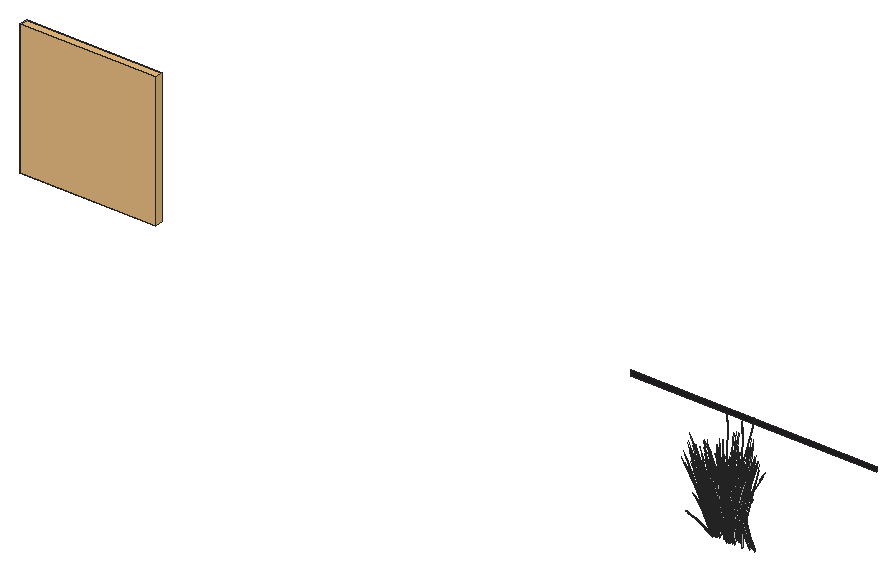
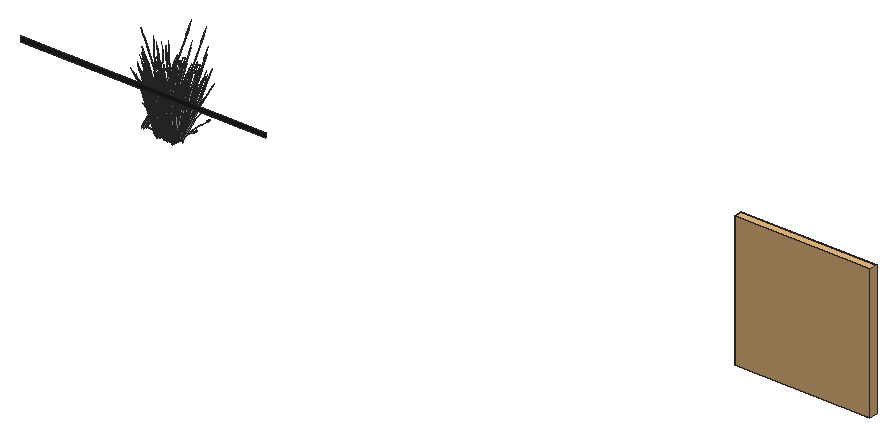
# SketchUp Ruby script. Lengths in inches.
U = 1.inch
M = Sketchup.active_model
def pt(a) = Geom::Point3d.new(a.map { |v| v * U })
def face(e, loops, mat)
  f = e.add_face(loops[0].map { |a| pt(a) })
  loops[1..].each { |l| e.add_face(l.map { |a| pt(a) }).erase! }
  f.material = f.back_material = mat if mat
  f
end
# faces: each face lists its corners as indices into pts; further lists are holes
def faces(e, pts, list, mat = nil) = list.each { |f| face(e, (f[0].is_a?(Array) ? f : [f]).map { |l| l.map { |i| pts[i] } }, mat) }
# xy, xz, yz: faces in a plane at the given z, y or x. An outline is a flat list of corners, or four numbers for a rectangle; further outlines are holes
def ring(l) = l.size == 4 ? [[l[0], l[1]], [l[2], l[1]], [l[2], l[3]], [l[0], l[3]]] : l.each_slice(2).to_a
def flat(e, list, mat, &to3) = list.each { |f| face(e, (f[0].is_a?(Array) ? f : [f]).map { |l| ring(l).map { |u, v| to3.(u, v) } }, mat) }
def xy(e, z, list, mat = nil) = flat(e, list, mat) { |x, y| [x, y, z] }
def xz(e, y, list, mat = nil) = flat(e, list, mat) { |x, z| [x, y, z] }
def yz(e, x, list, mat = nil) = flat(e, list, mat) { |y, z| [x, y, z] }
def lines(e, pts, list) = list.each { |a, b| e.add_line(pt(pts[a]), pt(pts[b])) }
# prism: a flat outline (further loops are holes) pulled along v
def prism(e, loops, v, mat = nil)
  f = face(e, loops, mat); d = Geom::Vector3d.new(v.map { |x| x * U })
  f.pushpull(f.normal.samedirection?(d) ? d.length : -d.length)
end
def box(e, o, s, mat = nil) = prism(e, [[o, [o[0] + s[0], o[1], o[2]], [o[0] + s[0], o[1] + s[1], o[2]], [o[0], o[1] + s[1], o[2]]]], [0, 0, s[2]], mat)
def at(x, y, z, deg = 0) = Geom::Transformation.translation(pt([x, y, z])) * Geom::Transformation.rotation(ORIGIN, Z_AXIS, deg.degrees)
def axes(o, x, y, z) = Geom::Transformation.new([*x, 0, *y, 0, *z, 0, *pt(o).to_a, 1])
def part(name) = M.definitions.add(name)
# library, detail: a bought-in or finely detailed component or shape, given as its bounding box
def library(name, o, s) = part(name).tap { |d| box(d.entities, o, s) }
def detail(e, o, s) = box(e.add_group.entities, o, s)
def put(e, d, t, mat = nil) = e.add_instance(d, t).tap { |i| i.material = mat if mat }
def group(e, t, mat = nil) = e.add_group.tap { |g| g.transformation = t; g.material = mat if mat }.entities
root = M.entities
M.materials.add("LightPink_Translucent").color = [144, 107, 117]
M.materials["LightPink_Translucent"].alpha = 0.75
M.materials.add("Marble_07_1K").color = [36, 34, 36]
c1 = library("mesh-163",[-551.08,-704.17,-20.03],[1929.24,1401.85,86.96])
c2 = part("Group11")
put(c2.entities,c1,at(0,0,0))
c3 = part("blade")
p = [[2.15,0.21,22],[0,0.17,0],[0.09,0.45,0],[2.18,0.31,22],[2.29,0.31,22],[0.38,0.45,0],
  [2.48,0.24,33],[2.49,0.24,33],[2.48,0.22,33]]
faces(c3.entities,p,[[0,1,2,3],[4,5,2,3],[6,3,4,7],[8,0,3,6]])
c4 = part("seeds")
p = [[0.3,-0.1,1.38],[-0.01,-0.03,1.59],[-0.01,-0.03,0.03],[0.14,-0.07,-0.07],[0.29,-0.03,3],[0.15,0.01,3.11]]
faces(c4.entities,p,[[0,1,2,3],[1,0,4,5]],"LightPink_Translucent")
c5 = part("blade with seeds")
put(c5.entities,c3,at(0,0,0))
put(c5.entities,c4,axes([2.4,0.25,30.99],[1.5799,-0.05474,1.17369],[-0.12525,1.92788,0.29478],[-0.07173,-0.02425,1.56792]))
xz(root,360,[[603,298,706,300]],"Marble_07_1K")
put(root,c2,axes([387.26,360.79,312.36],[-0.02948,0,0],[0,0,0.03987],[0,0.03937,0]))
put(root,c5,axes([657.47,336.1,267.22],[0.26985,-0.01293,1.42242],[-0.17902,0.56047,0.11501],[-0.38456,-0.03467,0.60807]))
put(root,c5,axes([657.58,337.08,267.22],[0.22574,-0.12077,1.42242],[0.19004,0.55807,0.11501],[-0.35439,0.12613,0.60807]))
put(root,c5,axes([658.875,336.5,266.77],[0.18493,-0.0826,1.46963],[0.06377,0.5767,0.11501],[-0.40056,0.07652,0.52526]))
put(root,c5,axes([656.89,336.89,267.91],[-0.10624,0.07413,1.45204],[0.00904,0.54162,-0.22964],[-0.24352,0.07044,0.11645]))
put(root,c5,axes([658.27,335.58,268.13],[-0.65035,-0.01375,-0.58968],[0.04368,-0.5789,0.07116],[-0.27552,-0.06109,0.83415]))
put(root,c5,axes([657.23,336.58,267.76],[-0.54068,-0.15928,-0.29394],[0.1577,-0.46469,0.37948],[-0.21769,0.04261,0.72609]))
put(root,c5,axes([655.71,337.43,267.91],[0.08303,0.01531,1.47228],[0.25685,0.50448,-0.13912],[-0.16996,0.13241,0.26054]))
put(root,c5,axes([657.6,336.8125,267.89],[-0.17625,0.51936,-0.42412],[-0.60429,-0.17802,-0.32852],[-0.2433,0.04762,0.81151]))
put(root,c5,axes([658.06,335.69,267.89],[-0.47241,0.37822,-0.42412],[-0.41372,-0.39954,-0.32852],[-0.24002,-0.05755,0.81151]))
put(root,c5,axes([657.39,334.63,267.91],[0.04823,0.05698,1.47228],[-0.23252,0.51221,-0.13912],[-0.23548,0.00371,0.26054]))
put(root,c5,axes([657.93,334.29,267.91],[-0.13998,-0.00403,1.45204],[-0.44565,0.40302,-0.22964],[-0.23779,-0.08235,0.11645]))
put(root,c5,axes([657.35,336.52,267.93],[0.18381,-0.5206,0.39842],[0.60429,0.17802,0.32852],[-0.23764,0.03129,0.82444]))
put(root,c5,axes([657.57,336.37,268.18],[0.32734,0.51701,-0.10093],[-0.58097,0.25407,-0.56021],[-0.24483,0.06821,0.85122]))
put(root,c5,axes([658.3,335.3,268.18],[-0.03484,0.58066,-0.10093],[-0.65957,-0.01587,-0.56021],[-0.25402,-0.04034,0.85122]))
put(root,c5,axes([657.88,335.34,267.76],[-0.37017,-0.35748,-0.29394],[0.42268,-0.3384,0.37948],[-0.21476,-0.05149,0.72609]))
put(root,c5,axes([657.31,336.38,267.93],[-0.23895,-0.38931,0.05337],[0.43573,-0.19055,0.42015],[-0.19208,0.0376,0.64067]))
put(root,c5,axes([658.4,337.46,267.22],[0.1625,-0.17544,1.42242],[0.41029,0.47354,0.11501],[-0.28141,0.21565,0.60807]))
put(root,c5,axes([657.43,337.92,267.76],[-0.56631,0.0816,-0.29394],[-0.14954,-0.46647,0.37948],[-0.16229,0.12529,0.72609]))
put(root,c5,axes([657.5,337.82,267.93],[-0.16135,-0.52549,0.39842],[0.63294,-0.0912,0.32852],[-0.18654,0.12359,0.82444]))
put(root,c5,axes([657.83,335.2,268.23],[0.53728,-0.42137,0.44623],[0.46337,0.44748,0.36794],[-0.25207,-0.07773,0.92337]))
put(root,c5,axes([657.375,337.72,267.93],[-0.44663,-0.24013,0.05337],[0.26003,-0.34195,0.42015],[-0.14319,0.11055,0.64067]))
put(root,c5,axes([658.28,337.89,267.22],[0.12114,-0.19625,1.42242],[0.50818,0.40613,0.11501],[-0.22925,0.25313,0.60807]))
put(root,c5,axes([657.8,336.53,268.19],[0.54068,0.15928,0.29394],[-0.1577,0.46469,-0.37948],[-0.21769,0.04261,0.72609]))
put(root,c5,axes([657.89,337.97,267.89],[0.16713,0.52135,-0.42412],[-0.63294,0.0912,-0.32852],[-0.18138,0.14003,0.81151]))
put(root,c5,axes([658.07,335.2,267.93],[0.03276,-0.43418,0.05337],[0.49468,0.0119,0.42015],[-0.18949,-0.04543,0.64067]))
put(root,c5,axes([656.9,338.91,267.91],[-0.01617,0.11299,1.45204],[0.45894,0.39307,-0.22964],[-0.12015,0.18588,0.11645]))
put(root,c5,axes([659.59,334.45,268.51],[-0.4342,0.54737,-0.11304],[-0.6288,-0.31535,-0.62743],[-0.21858,-0.15465,0.95337]))
put(root,c5,axes([658.41,335.52,268.19],[0.37017,0.35748,0.29394],[-0.42268,0.3384,-0.37948],[-0.21476,-0.05149,0.72609]))
put(root,c5,axes([657.59,337.6,268.18],[0.60181,0.31483,-0.10093],[-0.34671,0.45593,-0.56021],[-0.17003,0.15849,0.85122]))
put(root,c5,axes([656.6,338.97,268.6875],[0.5741,0.15241,-0.05385],[-0.1766,0.46909,-0.24415],[-0.0939,0.07122,0.8053]))
put(root,c5,axes([657.89,337.64,268.19],[0.56631,-0.0816,0.29394],[0.14954,0.46647,-0.37948],[-0.16229,0.12529,0.72609]))
put(root,c5,axes([658.42,338.88,267.93],[-0.46327,-0.38957,0.39842],[0.49199,-0.33598,0.32852],[-0.08546,0.18277,0.82444]))
put(root,c5,axes([658.25,338.84,267.93],[-0.53464,-0.0266,0.05337],[0.01466,-0.40172,0.42015],[-0.05594,0.15388,0.64067]))
put(root,c5,axes([658.42,339,267.76],[-0.4402,0.30062,-0.29394],[-0.41671,-0.34326,0.37948],[-0.0634,0.1744,0.72609]))
put(root,c5,axes([659.55,334.9,268.19],[0.10048,0.4599,0.29394],[-0.5744,0.12144,-0.37948],[-0.15428,-0.13179,0.72609]))
put(root,c5,axes([656.85,340.07,267.91],[0.07381,-0.03447,1.47228],[0.61004,0.22929,-0.13912],[-0.01434,0.19091,0.26054]))
put(root,c5,axes([660.73,338.02,266.76],[0.56221,0.23024,1.25546],[-0.55078,0.49601,0.49647],[-0.2467,-0.29398,1.05249]))
put(root,c5,axes([658.72,338.68,268.43],[-0.01693,0.52814,-0.65454],[-0.71285,-0.03547,0.07899],[-0.07523,0.22375,0.92591]))
put(root,c5,axes([664.17,335.5625,267.22],[0.26985,-0.01293,1.42242],[-0.17902,0.56047,0.11501],[-0.38456,-0.03467,0.60807]))
put(root,c5,axes([658.48,339.42,266.79],[0.01429,-0.29475,1.28107],[0.64291,0.15569,0.17703],[-0.0557,0.31414,0.60492]))
put(root,c5,axes([658.86,338.86,268.15],[0.46573,0.38364,-0.47077],[-0.49199,0.33598,-0.36465],[-0.07086,0.19492,0.90078]))
put(root,c5,axes([658.65,338.57,268.19],[0.4402,-0.30062,0.29394],[0.41671,0.34326,-0.37948],[-0.0634,0.1744,0.72609]))
put(root,c5,axes([664.28,336.55,267.22],[0.22574,-0.12077,1.42242],[0.19004,0.55807,0.11501],[-0.35439,0.12613,0.60807]))
put(root,c5,axes([661.6,336.91,266.36],[-0.01777,-0.53759,1.17256],[0.80434,0.13935,0.49647],[-0.19024,0.29416,1.1068]))
put(root,c5,axes([658.37,338.65,268.48],[0.71502,0.02829,-0.11203],[-0.01954,0.53563,-0.62183],[-0.04967,0.20629,0.94486]))
put(root,c5,axes([665.58,335.96,266.77],[0.18493,-0.0826,1.46963],[0.06377,0.5767,0.11501],[-0.40056,0.07652,0.52526]))
put(root,c5,axes([659.39,338.3,267.22],[-0.01592,-0.21915,1.42242],[0.69015,0.14538,0.11501],[-0.04269,0.3123,0.60807]))
put(root,c5,axes([663.59,336.35,267.91],[-0.10624,0.07413,1.45204],[0.00904,0.54162,-0.22964],[-0.24352,0.07044,0.11645]))
put(root,c5,axes([664.98,335.04,268.13],[-0.65035,-0.01375,-0.58968],[0.04368,-0.5789,0.07116],[-0.27552,-0.06109,0.83415]))
put(root,c5,axes([663.93,336.04,267.76],[-0.54068,-0.15928,-0.29394],[0.1577,-0.46469,0.37948],[-0.21769,0.04261,0.72609]))
put(root,c5,axes([662.41,336.9,267.91],[0.08303,0.01531,1.47228],[0.25685,0.50448,-0.13912],[-0.16996,0.13241,0.26054]))
put(root,c5,axes([664.3,336.28,267.89],[-0.17625,0.51936,-0.42412],[-0.60429,-0.17802,-0.32852],[-0.2433,0.04762,0.81151]))
put(root,c5,axes([664.76,335.16,267.89],[-0.47241,0.37822,-0.42412],[-0.41372,-0.39954,-0.32852],[-0.24002,-0.05755,0.81151]))
put(root,c5,axes([659.88,339.43,268.2],[-0.64106,-0.14927,0.44225],[0.21921,-0.49074,0.36465],[0.03852,0.19299,0.91512]))
put(root,c5,axes([659.71,339.46,267.93],[-0.47939,0.19405,0.05337],[-0.23464,-0.35385,0.42015],[0.0463,0.15598,0.64067]))
put(root,c5,axes([664.09,334.1,267.91],[0.04823,0.05698,1.47228],[-0.23252,0.51221,-0.13912],[-0.23548,0.00371,0.26054]))
put(root,c5,axes([664.06,335.98,267.93],[0.18381,-0.5206,0.39842],[0.60429,0.17802,0.32852],[-0.23764,0.03129,0.82444]))
put(root,c5,axes([664.27,335.84,268.18],[0.32734,0.51701,-0.10093],[-0.58097,0.25407,-0.56021],[-0.24483,0.06821,0.85122]))
put(root,c5,axes([665.01,334.76,268.18],[-0.03484,0.58066,-0.10093],[-0.65957,-0.01587,-0.56021],[-0.25402,-0.04034,0.85122]))
put(root,c5,axes([664.59,334.8,267.76],[-0.37017,-0.35748,-0.29394],[0.42268,-0.3384,0.37948],[-0.21476,-0.05149,0.72609]))
put(root,c5,axes([664.01,335.85,267.93],[-0.23895,-0.38931,0.05337],[0.43573,-0.19055,0.42015],[-0.19208,0.0376,0.64067]))
put(root,c5,axes([665.11,336.92,267.22],[0.1625,-0.17544,1.42242],[0.41029,0.47354,0.11501],[-0.28141,0.21565,0.60807]))
put(root,c5,axes([664.13,337.38,267.76],[-0.56631,0.0816,-0.29394],[-0.14954,-0.46647,0.37948],[-0.16229,0.12529,0.72609]))
put(root,c5,axes([659.95,339.53,267.76],[-0.19614,0.43908,-0.29394],[-0.57222,-0.12807,0.37948],[0.05247,0.17678,0.72609]))
put(root,c5,axes([664.2,337.28,267.93],[-0.16135,-0.52549,0.39842],[0.63294,-0.0912,0.32852],[-0.18654,0.12359,0.82444]))
put(root,c5,axes([664.53,334.67,268.23],[0.53728,-0.42137,0.44623],[0.46337,0.44748,0.36794],[-0.25207,-0.07773,0.92337]))
put(root,c5,axes([664.08,337.18,267.93],[-0.44663,-0.24013,0.05337],[0.26003,-0.34195,0.42015],[-0.14319,0.11055,0.64067]))
put(root,c5,axes([659.54,340.31,267.91],[0.08247,0.09194,1.45204],[0.66552,0.03612,-0.22964],[0.06692,0.20277,0.11645]))
put(root,c5,axes([664.99,337.36,267.22],[0.12114,-0.19625,1.42242],[0.50818,0.40613,0.11501],[-0.22925,0.25313,0.60807]))
put(root,c5,axes([659.89,339.07,268.19],[0.19614,-0.43908,0.29394],[0.57222,0.12807,-0.37948],[0.05247,0.17678,0.72609]))
put(root,c5,axes([664.5,335.99,268.19],[0.54068,0.15928,0.29394],[-0.1577,0.46469,-0.37948],[-0.21769,0.04261,0.72609]))
put(root,c5,axes([664.6,337.4375,267.89],[0.16713,0.52135,-0.42412],[-0.63294,0.0912,-0.32852],[-0.18138,0.14003,0.81151]))
put(root,c5,axes([664.78,334.66,267.93],[0.03276,-0.43418,0.05337],[0.49468,0.0119,0.42015],[-0.18949,-0.04543,0.64067]))
put(root,c5,axes([663.61,338.375,267.91],[-0.01617,0.11299,1.45204],[0.45894,0.39307,-0.22964],[-0.12015,0.18588,0.11645]))
put(root,c5,axes([660.01,339.13,268.13],[0.31051,0.46426,-0.58968],[-0.63919,0.25873,0.07116],[0.07261,0.22432,0.83415]))
put(root,c5,axes([665.11,334.99,268.19],[0.37017,0.35748,0.29394],[-0.42268,0.3384,-0.37948],[-0.21476,-0.05149,0.72609]))
put(root,c5,axes([660.66,340.63,268.6875],[0.44958,-0.32756,-0.05385],[0.41194,0.35875,-0.24415],[0.029,0.10165,0.8053]))
put(root,c5,axes([664.3,337.0625,268.18],[0.60181,0.31483,-0.10093],[-0.34671,0.45593,-0.56021],[-0.17003,0.15849,0.85122]))
put(root,c5,axes([660.24,339.23,267.89],[0.63954,0.14313,-0.42412],[-0.21921,0.49074,-0.32852],[0.05864,0.19758,0.81151]))
put(root,c5,axes([659.69,339.25,268.18],[0.63664,-0.26583,-0.10093],[0.31286,0.47181,-0.56021],[0.084,0.19882,0.85122]))
put(root,c5,axes([663.31,338.43,268.6875],[0.5741,0.15241,-0.05385],[-0.1766,0.46909,-0.24415],[-0.0939,0.07122,0.8053]))
put(root,c5,axes([664.59,337.11,268.19],[0.56631,-0.0816,0.29394],[0.14954,0.46647,-0.37948],[-0.16229,0.12529,0.72609]))
put(root,c5,axes([662.16,335.32,268.19],[-0.4402,0.30062,0.29394],[-0.41671,-0.34326,-0.37948],[0.0634,-0.1744,0.72609]))
put(root,c5,axes([665.13,338.35,267.93],[-0.46327,-0.38957,0.39842],[0.49199,-0.33598,0.32852],[-0.08546,0.18277,0.82444]))
put(root,c5,axes([664.96,338.31,267.93],[-0.53464,-0.0266,0.05337],[0.01466,-0.40172,0.42015],[-0.05594,0.15388,0.64067]))
put(root,c5,axes([665.125,338.46,267.76],[-0.4402,0.30062,-0.29394],[-0.41671,-0.34326,0.37948],[-0.0634,0.1744,0.72609]))
put(root,c5,axes([661.48,339.31,267.93],[-0.64708,0.13103,0.39842],[-0.1123,-0.514,0.32852],[0.15218,0.15149,0.82444]))
put(root,c5,axes([661.35,339.41,267.93],[-0.29569,0.36271,0.05337],[-0.42107,-0.21117,0.42015],[0.13613,0.11629,0.64067]))
put(root,c5,axes([660.6,338.21,267.22],[-0.14872,-0.18332,1.42242],[0.6872,-0.15433,0.11501],[0.15531,0.28779,0.60807]))
put(root,c5,axes([666.26,334.37,268.19],[0.10048,0.4599,0.29394],[-0.5744,0.12144,-0.37948],[-0.15428,-0.13179,0.72609]))
put(root,c5,axes([663.56,339.53,267.91],[0.07381,-0.03447,1.47228],[0.61004,0.22929,-0.13912],[-0.01434,0.19091,0.26054]))
put(root,c5,axes([667.44,337.48,266.76],[0.56221,0.23024,1.25546],[-0.55078,0.49601,0.49647],[-0.2467,-0.29398,1.05249]))
put(root,c5,axes([665.42,338.14,268.43],[-0.01693,0.52814,-0.65454],[-0.71285,-0.03547,0.07899],[-0.07523,0.22375,0.92591]))
put(root,c5,axes([661.26,338.99,268.19],[-0.10048,-0.4599,0.29394],[0.5744,-0.12144,-0.37948],[0.15428,0.13179,0.72609]))
put(root,c5,axes([661.65,336.35,267.71],[-0.56218,-0.29666,1.14775],[0.59361,-0.46189,0.49522],[0.18138,0.27836,1.10941]))
put(root,c5,axes([660.7,339.64,267.91],[0.00193,-0.06913,1.47228],[0.55753,-0.30498,-0.13912],[0.19366,0.10886,0.26054]))
put(root,c5,axes([665.18,338.89,266.79],[0.01429,-0.29475,1.28107],[0.64291,0.15569,0.17703],[-0.0557,0.31414,0.60492]))
put(root,c5,axes([662.56,335.05,267.93],[0.53464,0.0266,0.05337],[-0.01466,0.40172,0.42015],[0.05594,-0.15388,0.64067]))
put(root,c5,axes([665.5625,338.32,268.15],[0.46573,0.38364,-0.47077],[-0.49199,0.33598,-0.36465],[-0.07086,0.19492,0.90078]))
put(root,c5,axes([665.36,338.04,268.19],[0.4402,-0.30062,0.29394],[0.41671,0.34326,-0.37948],[-0.0634,0.1744,0.72609]))
put(root,c5,axes([668.31,336.38,266.36],[-0.01777,-0.53759,1.17256],[0.80434,0.13935,0.49647],[-0.19024,0.29416,1.1068]))
put(root,c5,axes([662.92,336.25,268.19],[-0.56631,0.0816,0.29394],[-0.14954,-0.46647,-0.37948],[0.16229,-0.12529,0.72609]))
put(root,c5,axes([665.08,338.12,268.48],[0.71502,0.02829,-0.11203],[-0.01954,0.53563,-0.62183],[-0.04967,0.20629,0.94486]))
put(root,c5,axes([661.21,339.23,268.18],[0.38768,-0.48872,-0.10093],[0.56143,0.28156,-0.56021],[0.19516,0.13808,0.85122]))
put(root,c5,axes([666.09,337.77,267.22],[-0.01592,-0.21915,1.42242],[0.69015,0.14538,0.11501],[-0.04269,0.3123,0.60807]))
put(root,c5,axes([672.07,336.16,267.22],[0.26985,-0.01293,1.42242],[-0.17902,0.56047,0.11501],[-0.38456,-0.03467,0.60807]))
put(root,c5,axes([663.22,336.3,268.18],[-0.60181,-0.31483,-0.10093],[0.34671,-0.45593,-0.56021],[0.17003,-0.15849,0.85122]))
put(root,c5,axes([661.67,338.99,267.89],[0.64198,-0.13573,-0.42412],[0.1123,0.514,-0.32852],[0.17243,0.1473,0.81151]))
put(root,c5,axes([662.4,338.37,268.19],[-0.37017,-0.35748,0.29394],[0.42268,-0.3384,-0.37948],[0.21476,0.05149,0.72609]))
put(root,c5,axes([662.74,338.7,267.93],[-0.03276,0.43418,0.05337],[-0.49468,-0.0119,0.42015],[0.18949,0.04543,0.64067]))
put(root,c5,axes([662.79,338.56,267.93],[-0.47971,0.37622,0.39842],[-0.41372,-0.39954,0.32852],[0.22506,0.0694,0.82444]))
put(root,c5,axes([662.92,335.92,267.89],[-0.16713,-0.52135,-0.42412],[0.63294,-0.0912,-0.32852],[0.18138,-0.14003,0.81151]))
put(root,c5,axes([672.18,337.14,267.22],[0.22574,-0.12077,1.42242],[0.19004,0.55807,0.11501],[-0.35439,0.12613,0.60807]))
put(root,c5,axes([664.03,338.61,267.26],[-0.12452,-0.47997,-0.02898],[0.58854,-0.11034,-0.1314],[0.1229,0.03043,0.43341]))
put(root,c5,axes([663.01,337.37,268.19],[-0.54068,-0.15928,0.29394],[0.1577,-0.46469,-0.37948],[0.21769,-0.04261,0.72609]))
put(root,c5,axes([666.58,338.89,268.2],[-0.64106,-0.14927,0.44225],[0.21921,-0.49074,0.36465],[0.03852,0.19299,0.91512]))
put(root,c5,axes([673.48,336.56,266.77],[0.18493,-0.0826,1.46963],[0.06377,0.5767,0.11501],[-0.40056,0.07652,0.52526]))
put(root,c5,axes([666.41,338.93,267.93],[-0.47939,0.19405,0.05337],[-0.23464,-0.35385,0.42015],[0.0463,0.15598,0.64067]))
put(root,c5,axes([663.4375,336.18,267.93],[0.44663,0.24013,0.05337],[-0.26003,0.34195,0.42015],[0.14319,-0.11055,0.64067]))
put(root,c5,axes([663.3125,336.08,267.93],[0.16135,0.52549,0.39842],[-0.63294,0.0912,0.32852],[0.18654,-0.12359,0.82444]))
put(root,c5,axes([671.49,336.95,267.91],[-0.10624,0.07413,1.45204],[0.00904,0.54162,-0.22964],[-0.24352,0.07044,0.11645]))
put(root,c5,axes([672.88,335.63,268.13],[-0.65035,-0.01375,-0.58968],[0.04368,-0.5789,0.07116],[-0.27552,-0.06109,0.83415]))
put(root,c5,axes([661.6,337.64,267.22],[-0.24166,-0.09837,1.42242],[0.50011,-0.41269,0.11501],[0.3117,0.18617,0.60807]))
put(root,c5,axes([664.7,336.16,267.91],[-0.08498,-0.00434,1.47228],[-0.35287,-0.46464,-0.13912],[0.14171,-0.15278,0.26054]))
put(root,c5,axes([671.83,336.64,267.76],[-0.54068,-0.15928,-0.29394],[0.1577,-0.46469,0.37948],[-0.21769,0.04261,0.72609]))
put(root,c5,axes([663.39,335.98,267.76],[0.56631,-0.0816,-0.29394],[0.14954,0.46647,0.37948],[0.16229,-0.12529,0.72609]))
put(root,c5,axes([666.65,338.99,267.76],[-0.19614,0.43908,-0.29394],[-0.57222,-0.12807,0.37948],[0.05247,0.17678,0.72609]))
put(root,c5,axes([662.94,336.13,268.13],[0.33983,-0.45051,-0.58968],[0.59551,0.32017,0.07116],[0.20291,-0.16322,0.83415]))
put(root,c5,axes([663.5,337.51,267.93],[0.23895,0.38931,0.05337],[-0.43573,0.19055,0.42015],[0.19208,-0.0376,0.64067]))
put(root,c5,axes([662.93,338.56,267.76],[0.37017,0.35748,-0.29394],[-0.42268,0.3384,0.37948],[0.21476,0.05149,0.72609]))
put(root,c5,axes([662.51,338.6,268.18],[0.03484,-0.58066,-0.10093],[0.65957,0.01587,-0.56021],[0.25402,0.04034,0.85122]))
